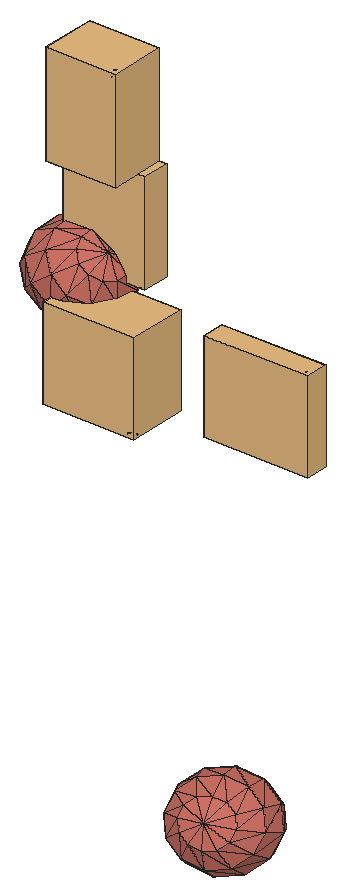
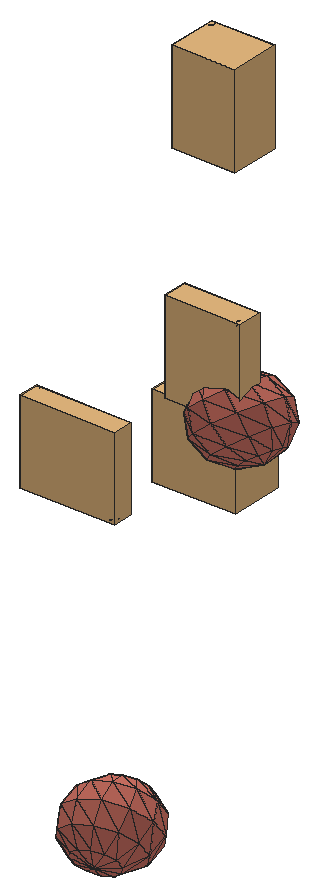
# SketchUp Ruby script. Lengths in inches.
U = 1.inch
M = Sketchup.active_model
def pt(a) = Geom::Point3d.new(a.map { |v| v * U })
def face(e, loops, mat)
  f = e.add_face(loops[0].map { |a| pt(a) })
  loops[1..].each { |l| e.add_face(l.map { |a| pt(a) }).erase! }
  f.material = f.back_material = mat if mat
  f
end
# faces: each face lists its corners as indices into pts; further lists are holes
def faces(e, pts, list, mat = nil) = list.each { |f| face(e, (f[0].is_a?(Array) ? f : [f]).map { |l| l.map { |i| pts[i] } }, mat) }
# xy, xz, yz: faces in a plane at the given z, y or x. An outline is a flat list of corners, or four numbers for a rectangle; further outlines are holes
def ring(l) = l.size == 4 ? [[l[0], l[1]], [l[2], l[1]], [l[2], l[3]], [l[0], l[3]]] : l.each_slice(2).to_a
def flat(e, list, mat, &to3) = list.each { |f| face(e, (f[0].is_a?(Array) ? f : [f]).map { |l| ring(l).map { |u, v| to3.(u, v) } }, mat) }
def xy(e, z, list, mat = nil) = flat(e, list, mat) { |x, y| [x, y, z] }
def xz(e, y, list, mat = nil) = flat(e, list, mat) { |x, z| [x, y, z] }
def yz(e, x, list, mat = nil) = flat(e, list, mat) { |y, z| [x, y, z] }
def lines(e, pts, list) = list.each { |a, b| e.add_line(pt(pts[a]), pt(pts[b])) }
# prism: a flat outline (further loops are holes) pulled along v
def prism(e, loops, v, mat = nil)
  f = face(e, loops, mat); d = Geom::Vector3d.new(v.map { |x| x * U })
  f.pushpull(f.normal.samedirection?(d) ? d.length : -d.length)
end
def box(e, o, s, mat = nil) = prism(e, [[o, [o[0] + s[0], o[1], o[2]], [o[0] + s[0], o[1] + s[1], o[2]], [o[0], o[1] + s[1], o[2]]]], [0, 0, s[2]], mat)
def at(x, y, z, deg = 0) = Geom::Transformation.translation(pt([x, y, z])) * Geom::Transformation.rotation(ORIGIN, Z_AXIS, deg.degrees)
def axes(o, x, y, z) = Geom::Transformation.new([*x, 0, *y, 0, *z, 0, *pt(o).to_a, 1])
def part(name) = M.definitions.add(name)
# library, detail: a bought-in or finely detailed component or shape, given as its bounding box
def library(name, o, s) = part(name).tap { |d| box(d.entities, o, s) }
def detail(e, o, s) = box(e.add_group.entities, o, s)
def put(e, d, t, mat = nil) = e.add_instance(d, t).tap { |i| i.material = mat if mat }
def group(e, t, mat = nil) = e.add_group.tap { |g| g.transformation = t; g.material = mat if mat }.entities
root = M.entities
M.materials.add("green").color = [174, 139, 102]
M.materials.add("vio").color = [206, 114, 100]
c1 = part("3DGeom~211_Defintion")
p = [[79.95,87.67,-500],[-17.63,-123.72,-495.48],[-148.11,-102.41,-480.17],[269.72,-13.2,-440.53],[-146.05,124.59,-473.48],[375.23,159.1,-301.875],
  [156.11,275.58,-370.54],[375.23,159.1,-301.875],[156.11,275.58,-370.54],[-110.49,-301.97,-358.2],[91.93,-181.96,-461.15],[-110.49,-301.97,-358.2],
  [-264.54,-123.72,-419.32],[-110.49,-301.97,-358.2],[-264.54,-123.72,-419.32],[-264.54,-123.72,-419.32],[-347.71,87.67,-368.09],[-104.85,318.21,-339.92],
  [-347.71,87.67,-368.09],[156.11,275.58,-370.54],[-104.85,318.21,-339.92],[151.22,-261.51,-386.375],[-110.49,-301.97,-358.2],[372.42,-150.98,-311.01],
  [372.42,-150.98,-311.01],[493.82,0,-152.32],[372.42,-150.98,-311.01],[269.72,-13.2,-440.53],[269.72,-13.2,-440.53],[375.23,159.1,-301.875],
  [-335.73,-181.96,-329.24],[-264.54,-123.72,-419.32],[-110.49,-301.97,-358.2],[-347.71,87.67,-368.09],[-264.54,-123.72,-419.32],[-335.73,-181.96,-329.24],
  [144.36,-341.07,-291.1875],[-110.49,-301.97,-358.2],[360.52,-288.77,-146.15],[360.52,-288.77,-146.15],[372.42,-150.98,-311.01],[380.21,288.77,-82.33],
  [156.11,275.58,-370.54],[190.4375,389.64,-141.8],[156.11,275.58,-370.54],[-104.85,318.21,-339.92],[380.21,288.77,-82.33],[156.11,275.58,-370.54],
  [190.4375,389.64,-141.8],[-471.01,-13.2,-212.05],[-337.71,275.58,-218.22],[-104.85,318.21,-339.92],[-347.71,87.67,-368.09],[-337.71,275.58,-218.22],
  [-43.26,-420.62,-140.25],[-173.74,-399.3,-124.94],[-110.49,-301.97,-358.2],[73.17,-399.3,-201.1],[-283.3,-341.07,-159.28],[144.36,-341.07,-291.1875],
  [-342.59,-261.51,-234.05],[-342.59,-261.51,-234.05],[-335.73,-181.96,-329.24],[-110.49,-301.97,-358.2],[-35.56,426.5625,-115.28],[-337.71,275.58,-218.22],
  [-342.59,-261.51,-234.05],[480.08,-159.1,38.05],[360.52,-288.77,-146.15],[482.9,150.98,47.19],[380.21,288.77,-82.33],[237.22,-389.64,9.88],
  [144.36,-341.07,-291.1875],[237.22,-389.64,9.88],[144.36,-341.07,-291.1875],[360.52,-288.77,-146.15],[-482.9,-150.98,-47.19],[-283.3,-341.07,-159.28],
  [-480.08,159.1,-38.05],[-237.22,389.64,-9.88],[-337.71,275.58,-218.22],[-237.22,389.64,-9.88],[35.56,-426.5625,115.28],[237.22,-389.64,9.88],
  [-380.21,-288.77,82.33],[-283.3,-341.07,-159.28],[-380.21,-288.77,82.33],[471.01,13.2,212.05],[337.71,-275.58,218.22],[237.22,-389.64,9.88],
  [283.3,341.07,159.28],[380.21,288.77,-82.33],[173.74,399.3,124.94],[-190.4375,-389.64,141.8],[-380.21,-288.77,82.33],[43.26,420.62,140.25],
  [342.59,261.51,234.05],[380.21,288.77,-82.33],[342.59,261.51,234.05],[380.21,288.77,-82.33],[283.3,341.07,159.28],[-493.82,0,152.32],
  [-360.52,288.77,146.15],[-237.22,389.64,-9.88],[-360.52,288.77,146.15],[-73.17,399.3,201.1],[-360.52,288.77,146.15],[104.85,-318.21,339.92],
  [237.22,-389.64,9.88],[104.85,-318.21,339.92],[237.22,-389.64,9.88],[337.71,-275.58,218.22],[347.71,-87.67,368.09],[335.73,181.96,329.24],
  [335.73,181.96,329.24],[342.59,261.51,234.05],[-375.23,-159.1,301.875],[-190.4375,-389.64,141.8],[-375.23,-159.1,301.875],[-156.11,-275.58,370.54],
  [-156.11,-275.58,370.54],[104.85,-318.21,339.92],[110.49,301.97,358.2],[110.49,301.97,358.2],[110.49,301.97,358.2],[-375.23,-159.1,301.875],
  [-190.4375,-389.64,141.8],[-156.11,-275.58,370.54],[-360.52,288.77,146.15],[-372.42,150.98,311.01],[-144.36,341.07,291.1875],[-360.52,288.77,146.15],
  [-372.42,150.98,311.01],[-360.52,288.77,146.15],[-144.36,341.07,291.1875],[-372.42,150.98,311.01],[-375.23,-159.1,301.875],[342.59,261.51,234.05],
  [110.49,301.97,358.2],[-144.36,341.07,291.1875],[110.49,301.97,358.2],[264.54,123.72,419.32],[264.54,123.72,419.32],[335.73,181.96,329.24],
  [146.05,-124.59,473.48],[104.85,-318.21,339.92],[337.71,-275.58,218.22],[337.71,-275.58,218.22],[347.71,-87.67,368.09],[335.73,181.96,329.24],
  [342.59,261.51,234.05],[110.49,301.97,358.2],[-151.22,261.51,386.37],[-269.72,13.2,440.53],[-375.23,-159.1,301.875],[-156.11,-275.58,370.54],
  [-372.42,150.98,311.01],[-375.23,-159.1,301.875],[-269.72,13.2,440.53],[264.54,123.72,419.32],[-79.95,-87.67,500],[17.63,123.72,495.48],
  [148.11,102.41,480.17],[-91.93,181.96,461.15],[347.71,-87.67,368.09],[347.71,-87.67,368.09]]
faces(c1.entities,p,[[0,1,2],[3,1,0],[0,2,4],[5,3,0],[6,0,4],[7,0,8],[2,1,9],[1,10,11],
  [3,10,1],[12,2,13],[4,2,14],[4,15,16],[17,4,18],[19,4,20],[10,21,22],[23,21,10],
  [24,10,3],[25,26,27],[25,28,29],[30,31,32],[33,34,35],[21,36,37],[38,36,21],[39,21,40],
  [41,29,42],[43,44,45],[46,47,48],[33,35,49],[50,33,49],[51,52,53],[54,55,56],[57,54,56],
  [55,58,56],[59,57,56],[58,60,56],[61,62,63],[64,45,65],[43,45,64],[49,35,66],[67,68,26],
  [67,26,25],[69,25,29],[69,29,70],[71,57,72],[73,74,75],[76,66,77],[49,66,76],[50,49,78],
  [79,50,78],[64,80,81],[78,49,76],[82,54,57],[82,57,83],[84,58,55],[76,85,86],[87,67,25],
  [87,25,69],[88,89,68],[88,68,67],[90,91,43],[90,43,92],[92,43,64],[93,54,82],[93,55,54],
  [94,55,93],[95,64,81],[92,64,95],[96,69,97],[98,99,100],[101,76,86],[78,76,101],[102,78,101],
  [103,78,104],[105,81,106],[95,81,105],[107,82,108],[109,110,111],[112,88,67],[112,67,87],[113,87,69],
  [114,69,115],[116,86,117],[101,86,118],[119,93,82],[120,82,121],[92,95,122],[90,92,123],[95,105,124],
  [125,126,127],[128,101,129],[130,131,132],[105,133,134],[135,101,136],[137,90,138],[105,139,140],[141,112,87],
  [142,87,143],[144,145,146],[144,147,148],[149,150,151],[130,132,152],[130,152,151],[153,154,155],[156,157,158],
  [152,132,153],[159,149,151],[160,155,145],[160,145,144],[161,162,151],[162,159,151],[163,161,151],[152,163,151],
  [162,144,164],[162,165,159],[153,155,160],[152,153,163],[163,153,160],[163,160,161],[161,160,144],[161,144,162]],"vio")
c2 = library("3DGeom~47_Defintion",[-132.29,-500,-408.57],[264.58,1000,817.14])
c3 = part("3DGeom~48_Defintion")
p = [[-103.8,487.39,-408.57],[-132.29,492.93,-365.46],[-123.73,496.1875,-348.87],[-103.8,487.39,-408.57],[-131.22,489.88,-384.15],[-132.29,492.93,-365.46],
  [-103.8,487.39,-408.57],[-120.79,487.85,-399.93],[-131.22,489.88,-384.15],[-103.8,487.39,-408.57],[-123.73,496.1875,-348.87],[-107.82,498.77,-338.8125],
  [-103.8,487.39,-408.57],[-107.82,498.77,-338.8125],[-88.83,500,-338],[-103.8,487.39,-408.57],[-60.34,494.46,-381.11],[-68.9,491.2,-397.7],
  [-103.8,487.39,-408.57],[-68.9,491.2,-397.7],[-84.8125,488.61,-407.76],[-103.8,487.39,-408.57],[-71.84,499.54,-346.64],[-61.42,497.51,-362.41],
  [-103.8,487.39,-408.57],[-61.42,497.51,-362.41],[-60.34,494.46,-381.11],[-103.8,487.39,-408.57],[-88.83,500,-338],[-71.84,499.54,-346.64],
  [91.01,-500,353.89],[109.71,-496.86,353.62],[124.82,-489.05,360.72],[62.5,-490.37,374.27],[91.01,-500,353.89],[67.8125,-469.79,401.48],
  [91.01,-500,353.89],[62.5,-490.37,374.27],[73.73,-497.625,361.44],[91.01,-500,353.89],[101.625,-458.84,408.31],[130.13,-468.47,387.93],
  [91.01,-500,353.89],[124.82,-489.05,360.72],[91.01,-500,353.89],[130.13,-468.47,387.93],[130.13,-468.47,387.93],[124.82,-489.05,360.72],
  [132.29,-478.66,373.28],[62.5,-490.37,374.27],[60.34,-480.18,388.92],[130.13,-468.47,387.93],[118.9,-461.21,400.75],[82.93,-461.98,408.57]]
faces(c3.entities,p,[[0,1,2],[3,4,5],[6,7,8],[9,10,11],[12,13,14],[15,16,17],[18,19,20],[21,22,23],
  [24,25,26],[27,28,29],[30,31,32],[33,34,35],[36,37,38],[35,39,40],[41,42,43],[40,44,45],
  [46,47,48],[49,35,50],[40,51,52],[35,40,53]],"green")
c4 = library("3DGeom~80_Defintion",[-319.18,-499.03,-500],[638.36,998.06,1000])
c5 = part("3DGeom~81_Defintion")
p = [[-260.82,484.9,-487.59],[-282.95,457.07,-500],[-298.58,446.97,-491.37],[-260.82,484.9,-487.59],[-269.125,470.95,-498.62],[-282.95,457.07,-500],
  [-260.82,484.9,-487.59],[-298.58,446.97,-491.37],[-311.84,443.35,-475.05],[-260.82,484.9,-487.59],[-311.84,443.35,-475.05],[-319.18,447.2,-455.39],
  [-260.82,484.9,-487.59],[-318.61,457.48,-437.68],[-260.82,484.9,-487.59],[-318.61,457.48,-437.68],[-310.3125,471.43,-426.66],[-260.82,484.9,-487.59],
  [-310.3125,471.43,-426.66],[-296.49,485.3125,-425.27],[-260.82,484.9,-487.59],[-296.49,485.3125,-425.27],[-280.85,495.42,-433.9],[-260.82,484.9,-487.59],
  [-280.85,495.42,-433.9],[-267.59,499.03,-450.23],[-260.82,484.9,-487.59],[-267.59,499.03,-450.23],[-260.26,495.18,-469.88],[291.93,-495.13,436.625],
  [252.8,-496.44,450.23],[271.18,-499.03,439.58],[291.93,-495.13,436.625],[319.18,-473.5,454.71],[252.8,-496.44,450.23],[319.18,-473.5,454.71],
  [291.93,-495.13,436.625],[309.5,-485.78,442.16],[252.8,-496.44,450.23],[319.18,-473.5,454.71],[240.91,-476.12,481.92],[252.8,-496.44,450.23],
  [240.91,-476.12,481.92],[241.72,-488.05,465.72],[240.91,-476.12,481.92],[319.18,-473.5,454.71],[268.15,-454.48,500],[319.18,-473.5,454.71],
  [307.29,-453.17,486.4],[319.18,-473.5,454.71],[318.36,-461.56,470.9],[307.29,-453.17,486.4],[240.91,-476.12,481.92],[250.59,-463.83,494.46],
  [307.29,-453.17,486.4],[288.91,-450.58,497.05]]
faces(c5.entities,p,[[0,1,2],[3,4,5],[6,7,8],[9,10,11],[12,11,13],[14,15,16],[17,18,19],[20,21,22],
  [23,24,25],[26,27,28],[29,30,31],[32,33,34],[35,36,37],[38,39,40],[41,42,43],[44,45,46],
  [46,47,48],[49,50,51],[52,46,53],[46,54,55]],"green")
c6 = library("3DGeom~92_Defintion",[-269.59,-500,-344.14],[539.17,1000,688.28])
c7 = part("3DGeom~93_Defintion")
p = [[-217.33,-469.79,-343.43],[-251.16,-458.84,-336.67],[-234.01,-461.98,-344.14],[-217.33,-469.79,-343.43],[-220.35,-500,-290.57],[-251.16,-458.84,-336.67],
  [-201.93,-490.37,-320.375],[-201.93,-490.37,-320.375],[-217.33,-469.79,-343.43],[-205.59,-480.18,-334.73],[-269.59,-468.47,-306.87],[-251.16,-458.84,-336.67],
  [-269.59,-468.47,-306.87],[-264.18,-461.21,-323.03],[-220.35,-500,-290.57],[-201.93,-490.37,-320.375],[-207.33,-497.625,-304.21],[-254.18,-489.05,-283.82],
  [-269.59,-468.47,-306.87],[-254.18,-489.05,-283.82],[-265.93,-478.66,-292.52],[-220.35,-500,-290.57],[-237.5,-496.86,-283.11],[-254.18,-489.05,-283.82],
  [253.72,487.39,337.56],[230.5,498.77,271.66],[212.66,500,278.24],[253.72,487.39,337.56],[249.06,496.1875,274.79],[230.5,498.77,271.66],
  [253.72,487.39,337.56],[263.36,492.93,286.79],[249.06,496.1875,274.79],[253.72,487.39,337.56],[212.66,500,278.24],[200.33,499.54,292.76],
  [253.72,487.39,337.56],[269.58,489.88,304.45],[263.36,492.93,286.79],[253.72,487.39,337.56],[200.33,499.54,292.76],[196.8,497.51,311.34],
  [253.72,487.39,337.56],[266.06,487.85,323.03],[269.58,489.88,304.45],[253.72,487.39,337.56],[196.8,497.51,311.34],[203.02,494.46,329],
  [253.72,487.39,337.56],[203.02,494.46,329],[217.33,491.2,341.01],[253.72,487.39,337.56],[217.33,491.2,341.01],[235.89,488.61,344.14]]
faces(c7.entities,p,[[0,1,2],[3,4,5],[6,4,3],[7,8,9],[5,4,10],[11,12,13],[14,15,16],[10,4,17],
  [18,19,20],[21,22,23],[24,25,26],[27,28,29],[30,31,32],[33,34,35],[36,37,38],[39,40,41],
  [42,43,44],[45,46,47],[48,49,50],[51,52,53]],"green")
c8 = part("3DGeom~214_Defintion")
p = [[-289.85,-175.69,-352.13],[-81.66,-101.43,-479.48],[-0.05,-263.22,-393.3125],[242.66,-186.82,-378.86],[-0.05,-263.22,-393.3125],[148.41,0,-478.35],
  [-356.86,-82.28,-337.79],[-289.85,-175.69,-352.13],[-356.86,-82.28,-337.79],[-197.72,60.36,-454.64],[420.34,-60.36,-262.88],[338.72,101.43,-349.05],
  [420.34,-60.36,-262.88],[14.41,186.82,-449.67],[-425.79,-13.9,-263.21],[-356.86,-82.28,-337.79],[-425.79,-13.9,-263.21],[-317.11,178.79,-325.46],
  [222.67,263.22,-324.21],[-123.46,323.58,-300.5],[-242.73,-269.1,-302.38],[-0.05,-263.22,-393.3125],[25.26,-381.66,-219.23],[-0.05,-263.22,-393.3125],
  [271.875,-323.58,-177.85],[25.26,-381.66,-219.23],[-0.05,-263.22,-393.3125],[271.875,-323.58,-177.85],[-289.85,-175.69,-352.13],[-0.05,-263.22,-393.3125],
  [-242.73,-269.1,-302.38],[242.66,-186.82,-378.86],[445.64,-178.79,-88.8],[271.875,-323.58,-177.85],[242.66,-186.82,-378.86],[420.34,-60.36,-262.88],
  [-289.85,-175.69,-352.13],[-242.73,-269.1,-302.38],[-420.38,-202.87,-130.43],[-356.86,-82.28,-337.79],[338.72,101.43,-349.05],[485.39,82.28,-76.47],
  [338.72,101.43,-349.05],[438.27,175.69,-126.22],[222.67,263.22,-324.21],[338.72,101.43,-349.05],[-425.79,-13.9,-263.21],[-478.1875,11.13,-148.36],
  [-317.11,178.79,-325.46],[-407.86,222.15,-126.54],[-317.11,178.79,-325.46],[-407.86,222.15,-126.54],[-123.46,323.58,-300.5],[-317.11,178.79,-325.46],
  [222.67,263.22,-324.21],[371.26,269.1,-111.88],[103.27,381.66,-195.03],[103.27,381.66,-195.03],[371.26,269.1,-111.88],[222.67,263.22,-324.21],
  [-242.73,-269.1,-302.38],[-228.125,-337.48,-201.88],[-228.125,-337.48,-201.88],[-407.86,222.15,-126.54],[-228.25,373.64,-70.82],[-123.46,323.58,-300.5],
  [103.27,381.66,-195.03],[-123.46,323.58,-300.5],[500,13.9,24.03],[-228.125,-337.48,-201.88],[-12.52,-425.01,-3.88],[228.25,-373.64,70.82],
  [271.875,-323.58,-177.85],[-228.125,-337.48,-201.88],[-249.9375,-362.51,-77.55],[-249.9375,-362.51,-77.55],[103.27,381.66,-195.03],[302.33,337.48,-37.3],
  [371.26,269.1,-111.88],[12.52,425.01,3.88],[103.27,381.66,-195.03],[103.27,381.66,-195.03],[271.875,-323.58,-177.85],[407.86,-222.15,126.54],
  [228.25,-373.64,70.82],[271.875,-323.58,-177.85],[-500,-13.9,-24.03],[-302.33,-337.48,37.3],[-371.26,-269.1,111.88],[-438.27,-175.69,126.22],
  [-485.39,-82.28,76.47],[-445.64,178.79,88.8],[-228.25,373.64,-70.82],[420.38,202.87,130.43],[302.33,337.48,-37.3],[478.1875,-11.13,148.36],
  [-249.9375,-362.51,-77.55],[-103.27,-381.66,195.03],[-249.9375,-362.51,-77.55],[-302.33,-337.48,37.3],[-271.875,323.58,177.85],[-228.25,373.64,-70.82],
  [-271.875,323.58,177.85],[302.33,337.48,-37.3],[249.9375,362.51,77.55],[249.9375,362.51,77.55],[123.46,-323.58,300.5],[123.46,-323.58,300.5],
  [-271.875,323.58,177.85],[-25.26,381.66,219.23],[-302.33,-337.48,37.3],[-222.67,-263.22,324.21],[-302.33,-337.48,37.3],[-222.67,-263.22,324.21],
  [-371.26,-269.1,111.88],[317.11,-178.79,325.46],[123.46,-323.58,300.5],[407.86,-222.15,126.54],[317.11,-178.79,325.46],[-420.34,60.36,262.88],
  [249.9375,362.51,77.55],[228.125,337.48,201.88],[228.125,337.48,201.88],[-338.72,-101.43,349.05],[-222.67,-263.22,324.21],[425.79,13.9,263.21],
  [317.11,-178.79,325.46],[425.79,13.9,263.21],[425.79,13.9,263.21],[356.86,82.28,337.79],[425.79,13.9,263.21],[289.85,175.69,352.13],
  [356.86,82.28,337.79],[242.73,269.1,302.38],[289.85,175.69,352.13],[228.125,337.48,201.88],[242.73,269.1,302.38],[-242.66,186.82,378.85],
  [-242.66,186.82,378.85],[-25.26,381.66,219.23],[-271.875,323.58,177.85],[-103.27,-381.66,195.03],[-14.41,-186.82,449.67],[-222.67,-263.22,324.21],
  [-103.27,-381.66,195.03],[123.46,-323.58,300.5],[0.05,263.22,393.3125],[0.05,263.22,393.3125],[242.73,269.1,302.38],[-242.66,186.82,378.85],
  [0.05,263.22,393.3125],[-25.26,381.66,219.23],[-338.72,-101.43,349.05],[-242.66,186.82,378.85],[-420.34,60.36,262.88],[317.11,-178.79,325.46],
  [425.79,13.9,263.21],[356.86,82.28,337.79],[197.71,-60.36,454.64],[81.66,101.43,479.48],[242.73,269.1,302.38],[289.85,175.69,352.13],
  [242.73,269.1,302.38],[-222.67,-263.22,324.21],[-148.41,0,478.35],[-338.72,-101.43,349.05],[-222.67,-263.22,324.21],[-338.72,-101.43,349.05],
  [-242.66,186.82,378.85],[-242.66,186.82,378.85]]
faces(c8.entities,p,[[0,1,2],[1,3,4],[1,5,3],[6,1,7],[8,9,1],[9,5,1],[5,10,3],[5,11,12],
  [9,13,5],[13,11,5],[14,9,15],[16,17,9],[17,13,9],[13,18,11],[17,19,13],[19,18,13],
  [20,21,22],[23,24,25],[26,3,27],[28,29,30],[31,32,33],[34,35,32],[36,37,38],[39,36,38],
  [40,41,35],[42,43,41],[44,43,45],[46,39,38],[47,48,46],[47,49,50],[51,52,53],[54,55,43],
  [19,56,18],[57,58,59],[60,22,61],[37,62,38],[63,64,65],[64,66,67],[47,46,38],[35,68,32],
  [35,41,68],[69,22,70],[22,71,70],[22,72,71],[73,70,74],[62,75,38],[76,77,78],[79,77,80],
  [64,79,81],[82,83,84],[85,32,83],[86,47,38],[86,49,47],[75,87,38],[87,88,38],[88,89,38],
  [90,86,38],[89,90,38],[86,91,49],[91,92,49],[41,43,93],[43,55,93],[55,94,93],[32,95,83],
  [32,68,95],[96,70,97],[98,97,99],[68,41,93],[91,100,101],[102,79,64],[103,104,93],[79,105,77],
  [90,91,86],[70,106,97],[70,71,107],[108,109,79],[109,105,79],[95,68,93],[110,97,111],[112,113,114],
  [71,115,116],[71,117,118],[89,119,90],[90,119,91],[120,121,93],[109,122,105],[119,100,91],[88,123,89],
  [88,124,123],[89,123,119],[83,125,126],[83,95,127],[128,95,93],[129,130,93],[131,132,93],[133,134,93],
  [135,136,93],[119,137,100],[138,139,140],[141,142,143],[144,145,142],[146,122,109],[147,148,122],[149,150,151],
  [152,153,154],[155,156,157],[145,158,142],[145,155,158],[159,160,150],[159,161,162],[163,164,165],[166,142,164],
  [155,157,158],[158,157,161],[167,164,168],[158,161,159],[164,150,169],[164,159,150],[142,159,164],[142,158,159]],"vio")
c9 = library("3DGeom~59_Defintion",[-108.27,-437.54,-500],[216.54,875.08,1000])
c10 = part("3DGeom~60_Defintion")
p = [[-48.9,-398.48,-495.36],[-85.15,-397.34,-497.61],[-66.68,-395.0625,-500],[-105.49,-415.16,-476],[-99.36,-404.6875,-488.82],[-85.15,-397.34,-497.61],
  [-105.49,-415.16,-476],[-85.15,-397.34,-497.61],[-32.98,-417.45,-471.51],[-105.49,-415.16,-476],[-32.98,-417.45,-471.51],[-36.5625,-406.68,-484.93],
  [-53.33,-435.27,-449.91],[-105.49,-415.16,-476],[-32.98,-417.45,-471.51],[-89.58,-434.125,-452.15],[-105.49,-415.16,-476],[-53.33,-435.27,-449.91],
  [-105.49,-415.16,-476],[-89.58,-434.125,-452.15],[-101.92,-425.93,-462.58],[-53.33,-435.27,-449.91],[-32.98,-417.45,-471.51],[-39.12,-427.92,-458.69],
  [-89.58,-434.125,-452.15],[-53.33,-435.27,-449.91],[-71.8,-437.54,-447.51],[44.63,425.16,482.47],[105.29,413.34,449.94],[94.58,425.52,444.15],
  [44.63,425.16,482.47],[94.58,425.52,444.15],[79.01,434.375,445.83],[44.63,425.16,482.47],[79.01,434.375,445.83],[62.76,437.54,454.55],
  [44.63,425.16,482.47],[108.27,401.11,461.67],[105.29,413.34,449.94],[44.63,425.16,482.47],[62.76,437.54,454.55],[50.17,434.17,467.96],
  [44.63,425.16,482.47],[102.73,392.1,476.1875],[108.27,401.11,461.67],[44.63,425.16,482.47],[90.15,388.73,489.6],[102.73,392.1,476.1875],
  [44.63,425.16,482.47],[73.89,391.89,498.32],[90.15,388.73,489.6],[44.63,425.16,482.47],[58.33,400.75,500],[73.89,391.89,498.32],
  [44.63,425.16,482.47],[47.61,412.93,494.2]]
faces(c10.entities,p,[[0,1,2],[3,4,5],[0,6,7],[8,9,0],[10,0,11],[12,13,14],[15,16,17],[18,19,20],
  [21,22,23],[24,25,26],[27,28,29],[30,31,32],[33,34,35],[36,37,38],[39,40,41],[42,43,44],
  [45,46,47],[48,49,50],[51,52,53],[54,55,52]],"green")
g1 = group(root,at(15.3125,134.49,26.21))
put(g1,c1,axes([-1.43,0.29,11.48],[0,0.00038,0],[0,0,-0.00038],[-0.00038,0,0]),"vio")
g2 = group(root,at(15.3125,134.49,26.21))
put(g2,c2,axes([-1.33,0.32,11.7],[0,0.0004,0],[0,0,-0.0004],[-0.0004,0,0]),"green")
put(g2,c3,axes([-1.33,0.32,11.7],[0,0.0004,0],[0,0,-0.0004],[-0.0004,0,0]),"green")
g3 = group(root,at(15.3125,134.49,26.21))
put(g3,c4,axes([-1.23,0.18,11.28],[0,0.00036,0],[0,0,-0.00036],[-0.00036,0,0]),"green")
put(g3,c5,axes([-1.23,0.18,11.28],[0,0.00036,0],[0,0,-0.00036],[-0.00036,0,0]),"green")
g4 = group(root,at(15.3125,134.49,26.21))
put(g4,c6,axes([-1.01,-0.14,12.39],[0,0.0004,0],[0,0,-0.0004],[-0.0004,0,0]),"green")
put(g4,c7,axes([-1.01,-0.14,12.39],[0,0.0004,0],[0,0,-0.0004],[-0.0004,0,0]),"green")
g5 = group(root,at(15.3125,134.49,26.21))
put(g5,c8,axes([-0.88,0.3,9.71],[0,0.00039,0],[0,0,-0.00039],[-0.00039,0,0]),"vio")
g6 = group(root,at(15.3125,134.49,26.21))
put(g6,c9,axes([-0.81,0.41,11.17],[0,0.00041,0],[0,0,-0.00041],[-0.00041,0,0]),"green")
put(g6,c10,axes([-0.81,0.41,11.17],[0,0.00041,0],[0,0,-0.00041],[-0.00041,0,0]),"green")
